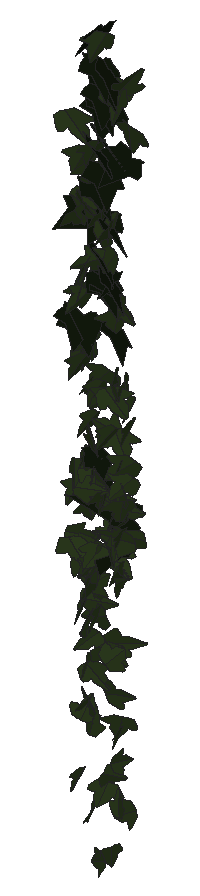
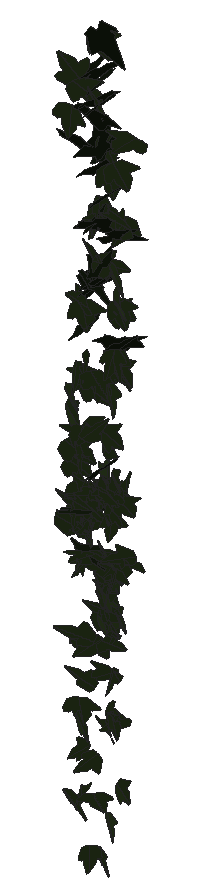
# SketchUp Ruby script. Lengths in inches.
U = 1.inch
M = Sketchup.active_model
def pt(a) = Geom::Point3d.new(a.map { |v| v * U })
def face(e, loops, mat)
  f = e.add_face(loops[0].map { |a| pt(a) })
  loops[1..].each { |l| e.add_face(l.map { |a| pt(a) }).erase! }
  f.material = f.back_material = mat if mat
  f
end
# faces: each face lists its corners as indices into pts; further lists are holes
def faces(e, pts, list, mat = nil) = list.each { |f| face(e, (f[0].is_a?(Array) ? f : [f]).map { |l| l.map { |i| pts[i] } }, mat) }
# xy, xz, yz: faces in a plane at the given z, y or x. An outline is a flat list of corners, or four numbers for a rectangle; further outlines are holes
def ring(l) = l.size == 4 ? [[l[0], l[1]], [l[2], l[1]], [l[2], l[3]], [l[0], l[3]]] : l.each_slice(2).to_a
def flat(e, list, mat, &to3) = list.each { |f| face(e, (f[0].is_a?(Array) ? f : [f]).map { |l| ring(l).map { |u, v| to3.(u, v) } }, mat) }
def xy(e, z, list, mat = nil) = flat(e, list, mat) { |x, y| [x, y, z] }
def xz(e, y, list, mat = nil) = flat(e, list, mat) { |x, z| [x, y, z] }
def yz(e, x, list, mat = nil) = flat(e, list, mat) { |y, z| [x, y, z] }
def lines(e, pts, list) = list.each { |a, b| e.add_line(pt(pts[a]), pt(pts[b])) }
# prism: a flat outline (further loops are holes) pulled along v
def prism(e, loops, v, mat = nil)
  f = face(e, loops, mat); d = Geom::Vector3d.new(v.map { |x| x * U })
  f.pushpull(f.normal.samedirection?(d) ? d.length : -d.length)
end
def box(e, o, s, mat = nil) = prism(e, [[o, [o[0] + s[0], o[1], o[2]], [o[0] + s[0], o[1] + s[1], o[2]], [o[0], o[1] + s[1], o[2]]]], [0, 0, s[2]], mat)
def at(x, y, z, deg = 0) = Geom::Transformation.translation(pt([x, y, z])) * Geom::Transformation.rotation(ORIGIN, Z_AXIS, deg.degrees)
def axes(o, x, y, z) = Geom::Transformation.new([*x, 0, *y, 0, *z, 0, *pt(o).to_a, 1])
def part(name) = M.definitions.add(name)
# library, detail: a bought-in or finely detailed component or shape, given as its bounding box
def library(name, o, s) = part(name).tap { |d| box(d.entities, o, s) }
def detail(e, o, s) = box(e.add_group.entities, o, s)
def put(e, d, t, mat = nil) = e.add_instance(d, t).tap { |i| i.material = mat if mat }
def group(e, t, mat = nil) = e.add_group.tap { |g| g.transformation = t; g.material = mat if mat }.entities
root = M.entities
M.materials.add("1026 AP 7946 SUNNY SIDE UP").color = [254, 231, 186]
M.materials.add("efeu1").color = [18, 25, 13]
M.materials.add("efeu2").color = [43, 57, 29]
c1 = part("ivyleaf_9")
p = [[1.54,2.16,1.25],[1.36,2.04,1.19],[-0.21,0.99,0.68],[-0.71,1.11,0.82],[-0.85,0.86,0.67],[-0.8,0.17,0.21],
  [-0.9,-0.01,0.1],[-0.67,-0.16,-0.02],[-0.08,-0.08,-0.05],[-0.03,-0.6,-0.4],[0.65,-0.88,-0.66],[0.83,-0.6,-0.49],
  [1.29,-0.42,-0.43],[1.8125,-0.07,-0.26],[1.21,0.44,0.15]]
faces(c1.entities,p,[[0,1,2,3,4,5,6,7,8,9,10,11,12,13,14]],"efeu1")
c2 = part("ivyleaf_10")
p = [[0,0.5,-0.03],[-0.0625,2.02,-0.43],[-0.19,2.01,-0.46],[-0.54,1.05,-0.29],[-0.52,0.625,-0.18],[-0.83,0.76,-0.28],
  [-1.16,0.64,-0.33],[-1.15,0.33,-0.24],[-0.77,-0.39,0.02],[-0.3,-0.51,0.16],[0.04,-0.48,0.23],[-0.02,2.01,-0.4375],
  [-0.06,2.01,-0.43],[0.04,-0.49,0.23],[0.67,-0.49,0.14],[1.38,0.36,-0.2],[1.375,0.51,-0.24],[0.81,0.65,-0.19],
  [0.62,0.59,-0.15],[0.6,1.09,-0.28],[0.5,1.23,-0.31]]
faces(c2.entities,p,[[0,1,2,3,4,5,6,7,8,9,10],[11,12,0,13,14,15,16,17,18,19,20]],"efeu2")
put(root,c1,axes([101.05,212.57,261.21],[-0.12089,-0.23192,0.03133],[-0.00458,-0.03244,-0.25178],[0.36804,-0.07658,0.00716]),"1026 AP 7946 SUNNY SIDE UP")
put(root,c2,axes([101.14,212.43,257.5],[-0.12326,-0.14817,0.13233],[0.01346,-0.14163,-0.16268],[0.30892,-0.05295,0.05989]),"1026 AP 7946 SUNNY SIDE UP")
put(root,c1,axes([101.25,212.67,263.58],[-0.26954,-0.12389,0.14208],[-0.14875,-0.1042,-0.21706],[0.25167,-0.19428,0.02388]),"1026 AP 7946 SUNNY SIDE UP")
put(root,c2,axes([100.91,212.42,265.73],[0.29451,0.09772,0.14047],[0.20088,0.05441,-0.2122],[-0.18925,0.20982,-0.00663]),"1026 AP 7946 SUNNY SIDE UP")
put(root,c2,axes([101.1875,212.51,261.94],[-0.11685,-0.21496,0.04703],[-0.0077,-0.04785,-0.23433],[0.34586,-0.07369,0.01067]),"1026 AP 7946 SUNNY SIDE UP")
put(root,c2,axes([101.23,212.51,265.02],[-0.18203,-0.19614,0.09728],[-0.02885,-0.09902,-0.23291],[0.34184,-0.1128,0.03214]),"1026 AP 7946 SUNNY SIDE UP")
put(root,c2,axes([101,212.43,256.35],[0.04919,0.0303,0.20582],[0.15419,0.1743,-0.04206],[-0.27752,0.10221,0.01311]),"1026 AP 7946 SUNNY SIDE UP")
put(root,c2,axes([101.15,212.63,258.17],[0.13111,-0.17614,0.06828],[0.04409,-0.06116,-0.20112],[0.29319,0.08797,-0.00029]),"1026 AP 7946 SUNNY SIDE UP")
put(root,c2,axes([100.98,212.61,260.5],[0.17531,-0.06217,0.20195],[0.24291,-0.12249,-0.13101],[0.21427,0.18973,-0.01671]),"1026 AP 7946 SUNNY SIDE UP")
put(root,c2,axes([101.13,212.35,257.99],[0.0088,0.19461,-0.10202],[-0.00113,-0.10015,-0.20114],[-0.34414,0.00531,-0.00195]),"1026 AP 7946 SUNNY SIDE UP")
put(root,c2,axes([101.1,212.63,262.12],[0.18927,-0.15272,0.16333],[0.12433,-0.13969,-0.2002],[0.3241,0.14278,-0.01858]),"1026 AP 7946 SUNNY SIDE UP")
put(root,c2,axes([101.22,212.51,261.8125],[-0.0432,-0.13076,0.21657],[0.0191,-0.21271,-0.13544],[0.38981,-0.00407,0.03064]),"1026 AP 7946 SUNNY SIDE UP")
put(root,c2,axes([101.0625,212.35,256.19],[-0.2549,-0.12594,-0.08462],[0.23675,-0.08413,-0.14428],[0.08317,-0.14649,0.15138]),"1026 AP 7946 SUNNY SIDE UP")
put(root,c2,axes([101.18,212.29,263.72],[-0.14646,-0.17995,-0.13754],[0.10165,0.1157,-0.20803],[0.33634,-0.11333,0.00298]),"1026 AP 7946 SUNNY SIDE UP")
put(root,c2,axes([101.24,212.37,251.0625],[0.0351,-0.18249,0.08916],[0.0253,-0.08624,-0.18983],[0.31727,0.02706,0.00527]),"1026 AP 7946 SUNNY SIDE UP")
put(root,c2,axes([100.98,212.6,263.85],[-0.07112,-0.04618,-0.25026],[0.32501,-0.14215,-0.01265],[-0.21267,-0.2018,0.06436]),"1026 AP 7946 SUNNY SIDE UP")
put(root,c2,axes([101.33,212.46,260.78],[0.2357,-0.09627,-0.14982],[-0.10355,0.14561,-0.16901],[0.25316,0.14919,0.07036]),"1026 AP 7946 SUNNY SIDE UP")
put(root,c1,axes([101.17,212.55,261.24],[-0.17214,-0.19654,-0.10592],[0.10387,0.07927,-0.23061],[0.3321,-0.12667,0.01722]),"1026 AP 7946 SUNNY SIDE UP")
put(root,c2,axes([101.31,212.41,255.78],[-0.0018,-0.04785,-0.2047],[-0.01523,0.19823,-0.04803],[0.3206,0.00915,-0.00343]),"1026 AP 7946 SUNNY SIDE UP")
put(root,c2,axes([101.33,212.33,260.46],[-0.05595,-0.21704,0.10373],[-0.02116,-0.10107,-0.22715],[0.37643,-0.03794,0.00265]),"1026 AP 7946 SUNNY SIDE UP")
put(root,c2,axes([101.32,212.47,262.62],[0.13992,-0.22095,0.03148],[0.00396,-0.03325,-0.24537],[0.35098,0.08846,-0.00978]),"1026 AP 7946 SUNNY SIDE UP")
put(root,c2,axes([101.34,212.47,252.66],[-0.00206,-0.20937,-0.02425],[-0.00385,0.02236,-0.21555],[0.33106,-0.00104,-0.00266]),"1026 AP 7946 SUNNY SIDE UP")
put(root,c2,axes([101.3,212.49,260.82],[-0.12068,-0.21718,-0.10534],[0.09366,0.08544,-0.23535],[0.36479,-0.09378,0.02558]),"1026 AP 7946 SUNNY SIDE UP")
put(root,c2,axes([101.26,212.3,255.85],[0.05821,0.22807,0.04414],[0.01659,0.04038,-0.23776],[-0.36414,0.0383,-0.00378]),"1026 AP 7946 SUNNY SIDE UP")
put(root,c2,axes([101.11,212.48,256.17],[-0.14041,-0.0145,-0.19807],[0.29241,-0.06212,-0.08455],[-0.07961,-0.20261,0.0388]),"1026 AP 7946 SUNNY SIDE UP")
put(root,c2,axes([101.32,212.33,254.91],[0.14266,-0.18629,0.05449],[0.03187,-0.05012,-0.21373],[0.30329,0.09289,-0.00317]),"1026 AP 7946 SUNNY SIDE UP")
put(root,c2,axes([101.36,212.61,259.05],[0.00321,-0.17691,0.15984],[0.01579,-0.15596,-0.18306],[0.37071,0.00817,0.00641]),"1026 AP 7946 SUNNY SIDE UP")
put(root,c2,axes([101.13,212.5,263.75],[-0.10092,0.04309,0.24743],[0.33163,-0.1146,0.07866],[0.19221,0.22035,-0.00579]),"1026 AP 7946 SUNNY SIDE UP")
put(root,c2,axes([101.36,212.49,257.1],[-0.12315,-0.18481,-0.05392],[0.0471,0.04293,-0.20625],[0.29788,-0.08319,0.01032]),"1026 AP 7946 SUNNY SIDE UP")
put(root,c2,axes([101.41,212.47,259.96],[0.04759,-0.22766,-0.08068],[-0.0175,0.07622,-0.23614],[0.37749,0.03224,-0.00077]),"1026 AP 7946 SUNNY SIDE UP")
put(root,c2,axes([101.55,212.32,252.63],[-0.07135,0.0725,-0.19229],[-0.15998,0.15698,0.08902],[0.27188,0.1114,0.00192]),"1026 AP 7946 SUNNY SIDE UP")
put(root,c2,axes([101.33,212.33,252.41],[0.18877,0.1291,-0.10543],[0.09399,0.08483,0.18168],[0.24215,-0.13356,0.01167]),"1026 AP 7946 SUNNY SIDE UP")
put(root,c2,axes([101.4,212.38,253.58],[0.04648,-0.16732,-0.13896],[0.05638,0.13716,-0.16756],[0.33225,0.00013,0.04787]),"1026 AP 7946 SUNNY SIDE UP")
put(root,c2,axes([101.27,212.59,257.32],[0.24188,-0.06309,0.11966],[0.17074,-0.04227,-0.17152],[0.11938,0.18828,0.00287]),"1026 AP 7946 SUNNY SIDE UP")
put(root,c2,axes([101.49,212.21,254.48],[0.07309,-0.07686,0.2262],[-0.15041,0.19828,0.09334],[-0.33416,-0.10606,0.00746]),"1026 AP 7946 SUNNY SIDE UP")
put(root,c2,axes([101.43,212.56,255.41],[0.07263,-0.15967,0.14803],[0.0483,-0.14149,-0.17189],[0.33525,0.05498,-0.0073]),"1026 AP 7946 SUNNY SIDE UP")
put(root,c2,axes([101.5,212.43,264.81],[-0.14419,-0.24198,0.02136],[0.00025,-0.02369,-0.26658],[0.38207,-0.09131,0.00824]),"1026 AP 7946 SUNNY SIDE UP")
put(root,c2,axes([101.18,212.53,257.75],[-0.00626,0.01645,0.23785],[0.36258,-0.01875,0.00537],[0.02999,0.23006,-0.01521]),"1026 AP 7946 SUNNY SIDE UP")
put(root,c2,axes([101.36,212.59,256.01],[-0.34015,-0.0764,-0.08258],[0.17812,-0.10086,-0.18869],[0.04241,-0.18915,0.13015]),"1026 AP 7946 SUNNY SIDE UP")
put(root,c2,axes([101.51,212.39,250.29],[0.05397,-0.18728,-0.07645],[-0.03337,0.07042,-0.19558],[0.31438,0.03963,-0.00763]),"1026 AP 7946 SUNNY SIDE UP")
put(root,c2,axes([101.46,212.41,255.54],[0.04738,-0.16888,-0.12079],[0.03979,0.1197,-0.17163],[0.31995,0.01012,0.03923]),"1026 AP 7946 SUNNY SIDE UP")
put(root,c2,axes([101.58,212.4375,255.88],[-0.10743,-0.13926,0.13969],[-0.07489,-0.12822,-0.1602],[0.29721,-0.08265,0.01013]),"1026 AP 7946 SUNNY SIDE UP")
put(root,c2,axes([101.62,212.49,262.75],[-0.04949,-0.06975,0.23602],[-0.12754,-0.21473,-0.07995],[0.35494,-0.08689,0.00418]),"1026 AP 7946 SUNNY SIDE UP")
put(root,c2,axes([101.67,212.4,255.3],[-0.11675,0.08854,-0.19184],[-0.20441,0.13421,0.11961],[0.25258,0.14954,0.00812]),"1026 AP 7946 SUNNY SIDE UP")
put(root,c2,axes([101.57,212.39,254.24],[0.1367,0.09156,-0.16348],[-0.16583,-0.11933,-0.13072],[-0.23643,0.13663,-0.00284]),"1026 AP 7946 SUNNY SIDE UP")
put(root,c2,axes([101.76,212.4,254.75],[-0.15145,0.04352,0.19795],[-0.30665,0.00741,-0.10252],[-0.0413,-0.21459,0.0353]),"1026 AP 7946 SUNNY SIDE UP")
put(root,c2,axes([101.48,212.42,257.7],[0.17597,0.15278,-0.10172],[0.07773,0.08708,0.19532],[0.27605,-0.12191,0.00984]),"1026 AP 7946 SUNNY SIDE UP")
put(root,c1,axes([101.65,212.52,267.95],[-0.12558,0.1968,-0.17026],[0.08257,-0.15811,-0.21955],[-0.39673,-0.0952,0.0082]),"1026 AP 7946 SUNNY SIDE UP")
put(root,c2,axes([101.54,212.39,255.88],[0.1894,-0.16964,0.02001],[0.00178,-0.02415,-0.21406],[0.26866,0.11975,-0.01269]),"1026 AP 7946 SUNNY SIDE UP")
put(root,c2,axes([101.6,212.34,258.53],[-0.25513,0.17082,-0.03513],[-0.01995,0.03621,0.24239],[0.27348,0.162,-0.01509]),"1026 AP 7946 SUNNY SIDE UP")
put(root,c2,axes([101.37,212.52,256.11],[0.10325,-0.13544,-0.15429],[0.16673,-0.10998,0.15048],[-0.26916,-0.12008,0.03403]),"1026 AP 7946 SUNNY SIDE UP")
put(root,c2,axes([101.6,212.55,257.6],[0.33025,-0.09068,-0.05328],[-0.08741,-0.00017,-0.23462],[0.13846,0.21618,-0.02104]),"1026 AP 7946 SUNNY SIDE UP")
put(root,c2,axes([101.57,212.34,252.17],[0.2736,-0.11654,0.07643],[-0.07759,0.06014,0.21499],[-0.2035,-0.17962,0.02078]),"1026 AP 7946 SUNNY SIDE UP")
put(root,c1,axes([101.43,212.52,264.38],[0.0794,-0.23226,-0.05774],[0.00383,0.05644,-0.24411],[0.37519,0.04857,0.01471]),"1026 AP 7946 SUNNY SIDE UP")
put(root,c2,axes([101.76,212.55,260.18],[-0.29242,-0.05595,0.12415],[-0.1706,-0.05663,-0.19939],[0.12136,-0.21442,0.01884]),"1026 AP 7946 SUNNY SIDE UP")
put(root,c2,axes([101.52,212.48,257.97],[-0.03026,-0.09022,-0.21034],[0.04765,-0.20358,0.08877],[-0.347,-0.02009,0.03053]),"1026 AP 7946 SUNNY SIDE UP")
put(root,c2,axes([101.34,212.24,257.59],[0.07442,-0.07881,-0.19835],[0.31949,-0.02295,0.06114],[-0.06717,-0.1965,0.07106]),"1026 AP 7946 SUNNY SIDE UP")
put(root,c2,axes([101.66,212.32,265.4],[-0.07464,-0.23856,0.05116],[-0.01107,-0.05061,-0.25085],[0.38343,-0.0479,0.00272]),"1026 AP 7946 SUNNY SIDE UP")
put(root,c2,axes([101.58,212.47,255.24],[0.16811,-0.17936,0.05813],[-0.02974,0.0555,0.21509],[-0.29464,-0.10793,0.01146]),"1026 AP 7946 SUNNY SIDE UP")
put(root,c2,axes([101.66,212.41,256.19],[0.27714,0.07116,-0.09511],[-0.1213,-0.05523,-0.19504],[-0.13807,0.19135,-0.01956]),"1026 AP 7946 SUNNY SIDE UP")
put(root,c1,axes([101.67,212.65,263.73],[-0.25385,-0.18364,0.02079],[-0.00497,-0.02544,-0.25161],[0.29064,-0.16083,0.01386]),"1026 AP 7946 SUNNY SIDE UP")
put(root,c2,axes([101.64,212.54,257.68],[0.33012,-0.10368,-0.01762],[-0.03742,-0.01104,-0.24037],[0.16079,0.2103,-0.01977]),"1026 AP 7946 SUNNY SIDE UP")
put(root,c2,axes([101.5,212.4,255.91],[0.27898,-0.03618,0.09965],[0.14562,-0.03025,-0.18645],[0.07253,0.1999,-0.00894]),"1026 AP 7946 SUNNY SIDE UP")
put(root,c2,axes([101.67,212.42,259.94],[-0.05651,-0.19363,0.10784],[0.01807,-0.10867,-0.20154],[0.34646,-0.02591,0.0281]),"1026 AP 7946 SUNNY SIDE UP")
put(root,c1,axes([101.5,212.56,258.26],[0.08645,-0.23896,-0.05474],[-0.01773,0.05053,-0.25231],[0.38405,0.05612,0.00067]),"1026 AP 7946 SUNNY SIDE UP")
put(root,c2,axes([101.62,212.47,254.78],[0.08545,-0.15993,0.15037],[0.07169,-0.13962,-0.17482],[0.33381,0.07092,-0.00095]),"1026 AP 7946 SUNNY SIDE UP")
put(root,c2,axes([101.38,212.46,254.98],[0.0508,-0.03717,-0.21734],[0.33519,-0.0133,0.036],[-0.02981,-0.21281,0.03442]),"1026 AP 7946 SUNNY SIDE UP")
put(root,c2,axes([101.72,212.46,267.78],[-0.1547,-0.21834,0.10251],[-0.01,-0.10645,-0.24469],[0.37796,-0.09218,0.03548]),"1026 AP 7946 SUNNY SIDE UP")
put(root,c2,axes([101.9375,212.54,257.23],[-0.11906,0.02523,0.20497],[-0.31513,-0.00856,-0.07756],[-0.00144,-0.21258,0.02619]),"1026 AP 7946 SUNNY SIDE UP")
put(root,c2,axes([101.71,212.625,266.52],[0.2671,-0.19242,0.01558],[-0.00193,-0.02267,-0.26405],[0.30363,0.16913,-0.01538]),"1026 AP 7946 SUNNY SIDE UP")
put(root,c1,axes([101.57,212.57,266.39],[0.06889,-0.24553,-0.02136],[-0.01539,0.01789,-0.25675],[0.38697,0.04443,-0.00641]),"1026 AP 7946 SUNNY SIDE UP")
put(root,c1,axes([101.51,212.64,262.77],[0.08561,-0.19727,0.15571],[0.07148,-0.14538,-0.21163],[0.38527,0.07081,0.00467]),"1026 AP 7946 SUNNY SIDE UP")
put(root,c2,axes([101.71,212.58,250.8],[0.26045,0.10573,-0.0658],[-0.07024,-0.0494,-0.20199],[-0.18161,0.17074,-0.01624]),"1026 AP 7946 SUNNY SIDE UP")
put(root,c1,axes([101.61,212.53,267.15],[-0.03829,-0.25106,-0.02538],[0.00742,0.02286,-0.25971],[0.39638,-0.02468,0.00241]),"1026 AP 7946 SUNNY SIDE UP")
put(root,c1,axes([101.55,212.57,266.91],[0.13689,-0.2433,0.00006],[-0.0087,-0.00351,-0.26614],[0.38247,0.087,-0.00608]),"1026 AP 7946 SUNNY SIDE UP")
put(root,c2,axes([101.71,212.15,255.6],[-0.0335,-0.11202,-0.18904],[0.07242,0.17709,-0.11625],[0.32933,-0.05033,0.00634]),"1026 AP 7946 SUNNY SIDE UP")
put(root,c1,axes([101.52,212.53,265.56],[0.33023,-0.16816,-0.01035],[-0.02892,-0.00847,-0.27659],[0.26322,0.21004,-0.01741]),"1026 AP 7946 SUNNY SIDE UP")
put(root,c2,axes([101.86,212.25,249.32],[0.11109,-0.1054,-0.16796],[-0.1419,0.13506,-0.12993],[0.26938,0.11461,0.00082]),"1026 AP 7946 SUNNY SIDE UP")
put(root,c1,axes([101.95,212.45,262.3],[-0.21538,0.20028,0.01562],[-0.03573,0.0014,-0.24927],[-0.31366,-0.13769,0.01767]),"1026 AP 7946 SUNNY SIDE UP")
put(root,c1,axes([101.67,212.59,266.47],[-0.08135,-0.2418,0.03013],[-0.00194,-0.03104,-0.25487],[0.38324,-0.05149,0.0051]),"1026 AP 7946 SUNNY SIDE UP")
put(root,c2,axes([101.54,212.3,253.53],[0.20929,0.07628,0.14782],[0.21432,0.04757,-0.1565],[-0.13803,0.18952,-0.01885]),"1026 AP 7946 SUNNY SIDE UP")
put(root,c1,axes([101.74,212.64,266.19],[-0.33415,-0.08221,-0.12191],[0.1853,0.02072,-0.23365],[0.12931,-0.24212,0.01981]),"1026 AP 7946 SUNNY SIDE UP")
put(root,c1,axes([101.54,212.46,265.28],[0.11295,-0.20008,0.13082],[0.07654,-0.11862,-0.21964],[0.36566,0.08663,0.00557]),"1026 AP 7946 SUNNY SIDE UP")
put(root,c2,axes([101.83,212.625,258.88],[0.0406,0.15275,0.167],[-0.04164,-0.15905,0.15867],[0.34675,-0.03698,-0.0005]),"1026 AP 7946 SUNNY SIDE UP")
put(root,c2,axes([101.6,212.3,255.47],[0.23389,-0.07858,-0.12591],[0.18415,-0.03762,0.17216],[-0.13424,-0.18852,0.01679]),"1026 AP 7946 SUNNY SIDE UP")
put(root,c1,axes([101.67,212.45,262.36],[0.05661,-0.21986,-0.10449],[-0.04074,0.09719,-0.22876],[0.37772,0.04344,-0.00901]),"1026 AP 7946 SUNNY SIDE UP")
put(root,c2,axes([101.72,212.43,257.4375],[-0.03379,0.08047,-0.21334],[0.04987,-0.20528,-0.08657],[-0.34645,-0.0374,0.00834]),"1026 AP 7946 SUNNY SIDE UP")
put(root,c2,axes([101.83,212.27,263.93],[-0.03287,-0.22314,-0.09984],[0.017,0.09505,-0.23033],[0.38137,-0.02347,0.00166]),"1026 AP 7946 SUNNY SIDE UP")
put(root,c2,axes([101.83,212.35,257.56],[-0.06104,-0.21674,-0.02646],[0.0167,0.02293,-0.22661],[0.34256,-0.03974,0.00633]),"1026 AP 7946 SUNNY SIDE UP")
put(root,c2,axes([101.95,212.41,259.82],[-0.15293,-0.12826,0.14664],[-0.12204,-0.12047,-0.16631],[0.27638,-0.12416,0.0077]),"1026 AP 7946 SUNNY SIDE UP")
put(root,c1,axes([101.7,212.5625,262.28],[0.04774,-0.24285,-0.03211],[-0.01489,0.02883,-0.25189],[0.38443,0.03127,-0.00577]),"1026 AP 7946 SUNNY SIDE UP")
put(root,c2,axes([102.02,212.68,266.67],[-0.21977,-0.11303,0.18392],[-0.11624,-0.17514,-0.17425],[0.31217,-0.14479,0.0646]),"1026 AP 7946 SUNNY SIDE UP")
put(root,c1,axes([102.26,212.63,257.07],[-0.37534,0.1311,0.18307],[-0.35429,-0.1863,-0.13998],[0.08117,-0.20698,0.23556]),"1026 AP 7946 SUNNY SIDE UP")
put(root,c2,axes([101.91,212.5,249.47],[-0.12002,-0.19131,-0.03219],[0.03861,0.0226,-0.21155],[0.30208,-0.0789,0.01425]),"1026 AP 7946 SUNNY SIDE UP")
put(root,c1,axes([101.83,212.61,256.18],[-0.28545,-0.15266,-0.12431],[0.32331,-0.12875,-0.11786],[0.01241,-0.15724,0.21145]),"1026 AP 7946 SUNNY SIDE UP")
put(root,c2,axes([101.96,212.4375,258.97],[-0.0396,-0.16859,0.14339],[-0.01037,-0.14042,-0.17607],[0.34457,-0.0236,0.01118]),"1026 AP 7946 SUNNY SIDE UP")
put(root,c2,axes([101.98,212.42,262.94],[0.26259,-0.17478,-0.05353],[-0.06997,0.02788,-0.24853],[0.27758,0.17236,-0.01201]),"1026 AP 7946 SUNNY SIDE UP")
put(root,c1,axes([101.84,212.38,264.82],[-0.04877,-0.25825,0.01218],[-0.00052,-0.01335,-0.26803],[0.40661,-0.03099,0.00112]),"1026 AP 7946 SUNNY SIDE UP")
put(root,c1,axes([101.76,212.48,263.74],[0.20576,-0.21248,0.0005],[-0.01625,-0.00835,-0.25677],[0.33372,0.1306,-0.01282]),"1026 AP 7946 SUNNY SIDE UP")
put(root,c2,axes([101.98,212.42,256.65],[0.09495,0.20757,-0.0343],[-0.00927,0.03752,0.22232],[0.33073,-0.05854,0.01608]),"1026 AP 7946 SUNNY SIDE UP")
put(root,c2,axes([101.93,212.2,263.5],[0.05053,0.11364,-0.2646],[0.07506,0.25321,0.12274],[0.43615,-0.05674,0.00953]),"1026 AP 7946 SUNNY SIDE UP")
put(root,c1,axes([101.82,212.53,267.04],[0.06587,-0.23415,0.10942],[0.01029,-0.10795,-0.2454],[0.40502,0.04082,-0.01156]),"1026 AP 7946 SUNNY SIDE UP")
put(root,c2,axes([101.92,212.42,256.77],[-0.06226,0.14769,-0.14167],[0.0362,-0.13678,-0.15799],[-0.31614,-0.04475,0.00981]),"1026 AP 7946 SUNNY SIDE UP")
put(root,c2,axes([102.01,212.4,257.14],[0.12193,-0.1835,-0.07849],[-0.01883,0.07621,-0.204],[0.31123,0.0765,0.01841]),"1026 AP 7946 SUNNY SIDE UP")
put(root,c2,axes([101.81,212.61,256.17],[-0.30682,-0.13758,-0.12149],[0.29583,-0.10909,-0.1596],[0.05453,-0.18233,0.18225]),"1026 AP 7946 SUNNY SIDE UP")
put(root,c2,axes([102.04,212.22,263.67],[0.00374,-0.2183,-0.10612],[0.00438,0.10179,-0.22427],[0.37869,0.00098,0.00364]),"1026 AP 7946 SUNNY SIDE UP")
put(root,c2,axes([101.81,212.47,257.48],[-0.00892,-0.05289,-0.20966],[0.2921,0.09352,-0.02987],[0.15395,-0.18051,0.04453]),"1026 AP 7946 SUNNY SIDE UP")
put(root,c2,axes([101.89,212.3,254.07],[-0.20976,-0.09925,-0.16168],[0.22223,0.07,-0.16957],[0.18822,-0.19326,0.02004]),"1026 AP 7946 SUNNY SIDE UP")
put(root,c2,axes([102.09,212.49,261.62],[-0.22244,-0.19625,0.02402],[-0.004,-0.02823,-0.24895],[0.31094,-0.14076,0.01399]),"1026 AP 7946 SUNNY SIDE UP")
put(root,c1,axes([101.85,212.49,262.38],[0.13411,-0.2212,0.08207],[0.02056,-0.08148,-0.24414],[0.36979,0.08475,-0.01619]),"1026 AP 7946 SUNNY SIDE UP")
put(root,c2,axes([102.24,212.09,256.46],[-0.04846,0.04743,0.24615],[-0.25543,0.17511,-0.05644],[-0.28488,-0.16508,0.00873]),"1026 AP 7946 SUNNY SIDE UP")
put(root,c1,axes([101.97,212.58,261.21],[0.03515,-0.2322,0.08938],[0.02022,-0.08723,-0.24079],[0.38997,0.02546,0.00443]),"1026 AP 7946 SUNNY SIDE UP")
put(root,c2,axes([102.05,212.2,251.38],[-0.08494,-0.0959,-0.18893],[0.1537,0.1546,-0.11238],[0.28597,-0.11158,0.00428]),"1026 AP 7946 SUNNY SIDE UP")
put(root,c2,axes([102.26,212.18,260.22],[-0.07189,0.085,0.23549],[-0.20774,0.18627,-0.0977],[-0.32149,-0.13937,0.01047]),"1026 AP 7946 SUNNY SIDE UP")
put(root,c2,axes([102.19,212.46,252.3125],[0.09035,-0.21082,0.02582],[0.00235,-0.02681,-0.22519],[0.33405,0.05721,-0.0054]),"1026 AP 7946 SUNNY SIDE UP")
put(root,c2,axes([102.03,212.51,258.87],[0.29384,0.12822,0.07617],[0.10928,0.0278,-0.23276],[-0.20484,0.19876,-0.01491]),"1026 AP 7946 SUNNY SIDE UP")
put(root,c2,axes([102.19,212.52,258.42],[0.09904,-0.20503,-0.05268],[0.00596,0.05324,-0.2198],[0.33177,0.06025,0.01968]),"1026 AP 7946 SUNNY SIDE UP")
put(root,c2,axes([102.18,212.39,256.64],[0.10967,0.18674,-0.08194],[-0.03949,-0.07665,-0.20578],[-0.31737,0.07407,-0.00271]),"1026 AP 7946 SUNNY SIDE UP")
put(root,c2,axes([102.09,212.22,253.95],[0.14632,0.06875,-0.21718],[0.1643,0.18852,0.11175],[0.3082,-0.13314,0.04354]),"1026 AP 7946 SUNNY SIDE UP")
put(root,c2,axes([102.48,212.24,256.76],[0.0458,-0.01768,-0.24953],[-0.37526,0.04256,-0.03253],[0.06989,0.24011,-0.01115]),"1026 AP 7946 SUNNY SIDE UP")
put(root,c2,axes([102.11,212.47,266.63],[0.33418,-0.15075,0.11219],[0.11128,-0.08875,-0.26728],[0.27127,0.22212,-0.02855]),"1026 AP 7946 SUNNY SIDE UP")
put(root,c2,axes([102.1875,212.32,251.61],[0.00126,0.0228,0.21342],[-0.03757,0.20568,-0.02204],[-0.32535,-0.02366,0.00337]),"1026 AP 7946 SUNNY SIDE UP")
put(root,c2,axes([102.24,212.3,250.54],[0.00875,0.16466,-0.12369],[-0.00435,0.12109,0.17035],[0.32128,-0.00285,0.00567]),"1026 AP 7946 SUNNY SIDE UP")
put(root,c2,axes([102.37,212.34,257.65],[-0.07248,0.06103,-0.223],[-0.16242,0.19093,0.07911],[0.31472,0.11259,-0.01053]),"1026 AP 7946 SUNNY SIDE UP")
put(root,c2,axes([102.3,212.35,252.6],[-0.27458,-0.11475,0.03661],[-0.03252,-0.03421,-0.21475],[0.18637,-0.17502,0.01647]),"1026 AP 7946 SUNNY SIDE UP")
put(root,c2,axes([102.28,212.39,257.45],[-0.18977,-0.19124,0.00491],[0.00838,-0.01028,-0.2328],[0.30073,-0.12039,0.00959]),"1026 AP 7946 SUNNY SIDE UP")
put(root,c2,axes([101.97,212.59,261.77],[0.0803,0.01022,0.24363],[0.35634,-0.07179,-0.04765],[0.1072,0.23099,-0.02411]),"1026 AP 7946 SUNNY SIDE UP")
put(root,c2,axes([102.26,212.47,257.02],[-0.03044,-0.17063,-0.11568],[0.01475,0.11096,-0.17624],[0.32001,-0.02135,-0.00288]),"1026 AP 7946 SUNNY SIDE UP")
put(root,c2,axes([102.03,212.47,254.2],[-0.09678,-0.03111,0.22225],[0.25956,0.14002,0.07008],[-0.22424,0.1755,-0.0148]),"1026 AP 7946 SUNNY SIDE UP")
put(root,c2,axes([102.41,212.45,258.38],[-0.17653,-0.13072,0.18082],[-0.1423,-0.1528,-0.17701],[0.31435,-0.14257,0.02142]),"1026 AP 7946 SUNNY SIDE UP")
put(root,c2,axes([102.26,212.25,255.77],[0.05636,-0.07157,-0.2204],[0.0383,0.21618,-0.06917],[0.35204,-0.01206,0.04281]),"1026 AP 7946 SUNNY SIDE UP")
put(root,c2,axes([102.27,212.26,255.99],[-0.01872,-0.15146,-0.1535],[0.0281,0.14712,-0.15558],[0.33194,-0.021,0.00451]),"1026 AP 7946 SUNNY SIDE UP")
put(root,c2,axes([102.27,212.45,260.16],[0.05204,-0.21322,-0.12321],[0.0387,0.12179,-0.21816],[0.38152,0.01673,0.03893]),"1026 AP 7946 SUNNY SIDE UP")
put(root,c2,axes([102.12,212.18,259.98],[0.2094,0.17072,0.12267],[0.11879,0.09084,-0.2225],[-0.30404,0.15308,-0.00245]),"1026 AP 7946 SUNNY SIDE UP")
put(root,c2,axes([102.06,212.32,253.11],[-0.13285,0.00851,0.19313],[0.29161,0.03487,0.0847],[-0.04461,0.2026,-0.02147]),"1026 AP 7946 SUNNY SIDE UP")
put(root,c2,axes([102.42,212.47,250.54],[0.19762,-0.12632,-0.14736],[-0.18286,0.08401,-0.18213],[0.23684,0.17027,-0.01767]),"1026 AP 7946 SUNNY SIDE UP")
put(root,c1,axes([102.41,212.44,265.3],[-0.40506,-0.023,-0.04669],[0.07396,-0.02094,-0.26535],[0.02979,-0.2607,0.02389]),"1026 AP 7946 SUNNY SIDE UP")
put(root,c2,axes([102.02,212.58,257.1875],[0.08383,-0.05998,-0.21733],[0.32266,-0.06203,0.07135],[-0.12027,-0.20822,0.03992]),"1026 AP 7946 SUNNY SIDE UP")
put(root,c2,axes([102.39,212.44,257.99],[-0.17851,-0.11429,0.16713],[-0.05223,-0.17401,-0.15065],[0.30848,-0.09559,0.07121]),"1026 AP 7946 SUNNY SIDE UP")
put(root,c2,axes([102.21,212.51,266.76],[-0.09801,-0.24882,0.1021],[0.06977,0.09222,0.26405],[-0.41615,0.07406,0.02022]),"1026 AP 7946 SUNNY SIDE UP")
put(root,c2,axes([102.56,212.55,256.71],[-0.05836,0.00682,0.21312],[-0.3163,-0.05056,-0.03576],[0.07646,-0.20397,0.01472]),"1026 AP 7946 SUNNY SIDE UP")
put(root,c2,axes([102.31,212.64,259.67],[0.16632,-0.17487,0.06179],[0.02546,-0.06121,-0.21016],[0.29009,0.10563,-0.01698]),"1026 AP 7946 SUNNY SIDE UP")
put(root,c2,axes([102.4,212.52,265.9],[-0.37383,0.0766,0.03739],[-0.06125,-0.0042,-0.25683],[-0.11805,-0.2404,0.01485]),"1026 AP 7946 SUNNY SIDE UP")
put(root,c2,axes([102.35,212.32,256.9],[0.06834,-0.20768,0.04084],[0.00732,-0.04072,-0.21879],[0.33272,0.04355,-0.00357]),"1026 AP 7946 SUNNY SIDE UP")
put(root,c2,axes([102.37,212.54,259.25],[0.08992,-0.21678,0.07046],[0.02034,-0.06858,-0.23131],[0.35744,0.05844,-0.00456]),"1026 AP 7946 SUNNY SIDE UP")
